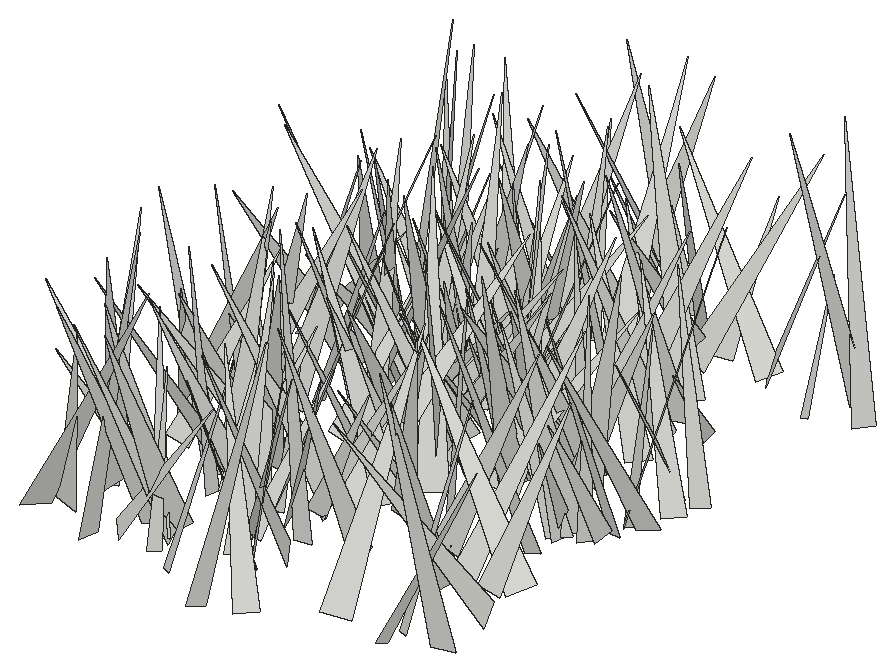
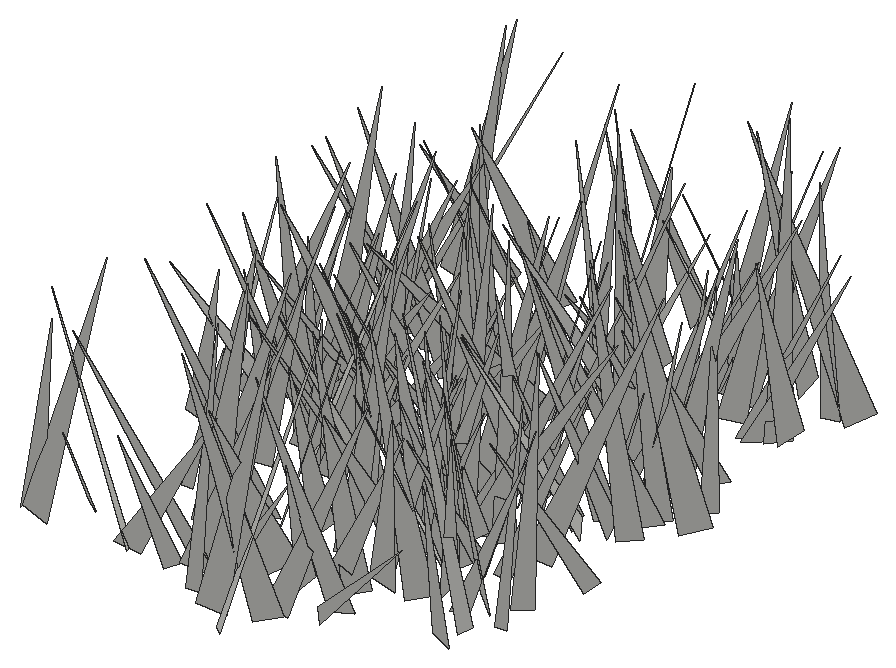
# SketchUp Ruby script. Lengths in inches.
U = 1.inch
M = Sketchup.active_model
def pt(a) = Geom::Point3d.new(a.map { |v| v * U })
def face(e, loops, mat)
  f = e.add_face(loops[0].map { |a| pt(a) })
  loops[1..].each { |l| e.add_face(l.map { |a| pt(a) }).erase! }
  f.material = f.back_material = mat if mat
  f
end
# faces: each face lists its corners as indices into pts; further lists are holes
def faces(e, pts, list, mat = nil) = list.each { |f| face(e, (f[0].is_a?(Array) ? f : [f]).map { |l| l.map { |i| pts[i] } }, mat) }
# xy, xz, yz: faces in a plane at the given z, y or x. An outline is a flat list of corners, or four numbers for a rectangle; further outlines are holes
def ring(l) = l.size == 4 ? [[l[0], l[1]], [l[2], l[1]], [l[2], l[3]], [l[0], l[3]]] : l.each_slice(2).to_a
def flat(e, list, mat, &to3) = list.each { |f| face(e, (f[0].is_a?(Array) ? f : [f]).map { |l| ring(l).map { |u, v| to3.(u, v) } }, mat) }
def xy(e, z, list, mat = nil) = flat(e, list, mat) { |x, y| [x, y, z] }
def xz(e, y, list, mat = nil) = flat(e, list, mat) { |x, z| [x, y, z] }
def yz(e, x, list, mat = nil) = flat(e, list, mat) { |y, z| [x, y, z] }
def lines(e, pts, list) = list.each { |a, b| e.add_line(pt(pts[a]), pt(pts[b])) }
# prism: a flat outline (further loops are holes) pulled along v
def prism(e, loops, v, mat = nil)
  f = face(e, loops, mat); d = Geom::Vector3d.new(v.map { |x| x * U })
  f.pushpull(f.normal.samedirection?(d) ? d.length : -d.length)
end
def box(e, o, s, mat = nil) = prism(e, [[o, [o[0] + s[0], o[1], o[2]], [o[0] + s[0], o[1] + s[1], o[2]], [o[0], o[1] + s[1], o[2]]]], [0, 0, s[2]], mat)
def at(x, y, z, deg = 0) = Geom::Transformation.translation(pt([x, y, z])) * Geom::Transformation.rotation(ORIGIN, Z_AXIS, deg.degrees)
def axes(o, x, y, z) = Geom::Transformation.new([*x, 0, *y, 0, *z, 0, *pt(o).to_a, 1])
def part(name) = M.definitions.add(name)
# library, detail: a bought-in or finely detailed component or shape, given as its bounding box
def library(name, o, s) = part(name).tap { |d| box(d.entities, o, s) }
def detail(e, o, s) = box(e.add_group.entities, o, s)
def put(e, d, t, mat = nil) = e.add_instance(d, t).tap { |i| i.material = mat if mat }
def group(e, t, mat = nil) = e.add_group.tap { |g| g.transformation = t; g.material = mat if mat }.entities
root = M.entities
c1 = part("fur_instance\#9")
p = [[0.8125,0,1.79],[0.67,-0.02,1.48],[0,-0.11,0],[0,0.11,0]]
faces(c1.entities,p,[[0,1,2,3]])
put(root,c1,axes([478.73,175.67,-21.66],[-5.72955,1.74546,0.28048],[1.75274,5.48455,1.67353],[-0.23061,-1.68113,5.75097]))
put(root,c1,axes([477.37,174.2,-21.66],[-6.45449,2.84921,1.13675],[2.42101,6.35763,-2.18855],[1.88385,1.59157,6.70736]))
put(root,c1,axes([478.21,201.08,-21.66],[1.19098,5.93826,0.851],[5.76454,-1.37303,1.51343],[-1.66049,-0.50738,5.86438]))
put(root,c1,axes([475.85,182.62,-21.66],[5.48383,-1.63022,0.30334],[-1.45467,-5.23263,-1.82362],[-0.79597,-1.66854,5.42259]))
put(root,c1,axes([476.59,198.27,-21.66],[-1.94792,-5.41513,0.85515],[-5.11405,2.12183,1.78705],[1.97517,0.15336,5.47032]))
put(root,c1,axes([479.69,182.78,-21.66],[-6.30755,-1.0303,0.95825],[-1.23667,6.15876,-1.51833],[0.67114,1.66527,6.20817]))
put(root,c1,axes([479.28,198.21,-21.66],[-4.32688,2.05759,1.06704],[2.30248,4.07514,1.47851],[0.2661,-1.80382,4.55737]))
put(root,c1,axes([478.76,196.84,-21.66],[4.06044,6.49572,1.60929],[6.19974,-4.35997,1.95581],[-2.5194,-0.26008,7.4065]))
put(root,c1,axes([479.375,175.64,-21.66],[-5.28354,-0.86585,0.73138],[-0.45173,4.80676,2.42722],[1.0395,-2.31209,4.77222]))
put(root,c1,axes([480.05,179.39,-21.66],[-1.59145,-6.67923,2.98055],[-7.18236,0.85085,-1.92829],[-1.38185,3.26993,6.58988]))
put(root,c1,axes([476.96,196.1,-21.66],[6.03542,-2.39463,0.80521],[-2.12324,-5.9379,-1.74415],[-1.3691,-1.34759,6.25448]))
put(root,c1,axes([475.61,192.22,-21.66],[3.92135,-2.35365,0.03406],[-2.05535,-3.39138,2.27856],[1.14733,1.96892,3.96545]))
put(root,c1,axes([477.05,171.45,-21.66],[-0.17668,-5.97479,1.5156],[-5.97573,0.53792,1.42395],[1.51188,1.4279,5.80532]))
put(root,c1,axes([479.55,191.72,-21.66],[4.2838,-6.03866,0.74714],[-5.20831,-4.11147,-3.36808],[-3.14598,-1.41597,6.59337]))
put(root,c1,axes([475.19,184.5,-21.66],[4.73655,-6.32836,0.37656],[-6.13582,-4.45802,2.25891],[1.59428,1.644,7.57499]))
put(root,c1,axes([481.03,193.74,-21.66],[-5.46466,-2.11839,0.66349],[-2.21236,5.05235,-2.09036],[-0.18243,2.18553,5.47545]))
put(root,c1,axes([477.65,174.89,-21.66],[7.83218,-2.47016,1.5817],[-2.12062,-7.88445,-1.81244],[-2.02643,-1.29626,8.00998]))
put(root,c1,axes([478.59,186.95,-21.66],[5.94248,2.0649,1.47313],[1.51819,-5.90154,2.14801],[-2.032,1.62942,5.91295]))
put(root,c1,axes([481.06,196.81,-21.66],[-6.67208,0.88571,0.68005],[0.61302,6.34873,-2.25421],[0.93335,2.16166,6.3419]))
put(root,c1,axes([477.32,180,-21.66],[-0.99691,5.86129,1.26655],[5.41282,1.43213,-2.36709],[2.58075,-0.73958,5.45394]))
put(root,c1,axes([479.28,183.15,-21.66],[5.03177,-2.92165,1.14225],[-2.20313,-4.82824,-2.64459],[-2.23316,-1.81978,5.18275]))
put(root,c1,axes([477.25,184.72,-21.66],[0.83878,-6.84447,1.51714],[-6.71971,-0.34936,2.13903],[1.99848,1.69801,6.55552]))
put(root,c1,axes([477.18,187.3,-21.66],[2.07111,-6.85146,1.31632],[-6.80663,-1.68294,1.94991],[1.53132,1.78604,6.88693]))
put(root,c1,axes([475.84,170.59,-21.66],[7.56022,-3.29271,0.03526],[-3.23696,-7.41517,1.59297],[0.60437,1.47429,8.09082]))
put(root,c1,axes([481.2,182.07,-21.66],[-6.30471,-1.37126,0.42808],[-1.05468,5.72683,2.8114],[0.97532,-2.67133,5.80738]))
put(root,c1,axes([484.07,190.01,-21.66],[-5.6206,-6.05261,0.8091],[-5.56666,4.62654,-4.06048],[-2.5102,3.29256,7.1929]))
put(root,c1,axes([479.79,194.22,-21.66],[4.40481,-2.70951,0.82389],[-1.71706,-3.76665,-3.20728],[-2.2521,-2.42766,4.05674]))
put(root,c1,axes([481.92,178.79,-21.66],[-0.45254,-7.13046,0.09555],[-6.72101,0.39447,-2.39372],[-2.38342,0.24148,6.7319]))
put(root,c1,axes([481.65,182.78,-21.66],[-4.16837,-0.36819,0.02902],[-0.35612,3.91965,-1.4217],[-0.09791,1.41863,3.93569]))
put(root,c1,axes([477.19,185.42,-21.66],[0.42432,7.03314,2.02201],[6.63788,0.48281,-3.07232],[3.08094,-2.00885,6.34082]))
put(root,c1,axes([479.92,169.64,-21.66],[-7.4216,0.05563,3.73189],[-0.80703,8.0859,-1.72548],[3.64401,1.90407,7.21845]))
put(root,c1,axes([482.03,176.91,-21.66],[-6.19983,-0.76734,1.02255],[-1.02443,6.01091,-1.70052],[0.76483,1.83095,6.01123]))
put(root,c1,axes([481.72,172.77,-21.66],[0.79588,-7.21699,0.96951],[-7.03929,-1.01213,-1.75565],[-1.86367,0.74092,7.04528]))
put(root,c1,axes([480.85,174.63,-21.66],[4.14575,-5.15062,1.64406],[-4.88287,-4.45639,-1.64839],[-2.32151,0.17524,6.40304]))
put(root,c1,axes([483.37,191.71,-21.66],[-7.87957,1.88276,1.17896],[2.17634,7.41366,2.70618],[0.44527,-2.91806,7.63603]))
put(root,c1,axes([480.29,187.55,-21.66],[4.99403,0.89918,1.35491],[0.3935,-4.91429,1.81096],[-1.5778,1.62046,4.74018]))
put(root,c1,axes([477.8125,199.6,-21.66],[8.03575,1.73258,0.69022],[1.85682,-7.7181,-2.24381],[-0.17451,-2.34107,7.90825]))
put(root,c1,axes([481.43,178.94,-21.66],[-6.63675,3.07759,1.929],[2.57186,6.8191,-2.03087],[2.56478,1.12578,7.02806]))
put(root,c1,axes([479.83,187.86,-21.66],[6.02604,4.35688,0.13616],[4.14402,-5.7981,2.12678],[-1.35204,1.64734,7.12547]))
put(root,c1,axes([479.25,186.46,-21.66],[0.24663,7.62872,2.41582],[7.70784,0.42293,-2.12242],[2.15005,-2.39126,7.33168]))
put(root,c1,axes([482.8125,171.75,-21.66],[0.07199,5.81915,0.58708],[5.58747,-0.24194,1.7129],[-1.72841,-0.53974,5.5618]))
put(root,c1,axes([484.52,202.88,-21.66],[-3.03964,-3.22245,0.08473],[-2.53096,2.3136,-2.80576],[-1.9964,1.97328,3.42802]))
put(root,c1,axes([482.71,178.54,-21.66],[-6.34287,-0.8603,1.40577],[-0.30586,6.10717,2.3574],[1.61949,-2.21602,5.95103]))
put(root,c1,axes([483.16,172.38,-21.66],[-6.61379,-2.13915,0.88077],[-1.88588,6.53057,1.69974],[1.33985,-1.36736,6.74011]))
put(root,c1,axes([482.19,194.6,-21.66],[-7.10447,-2.39928,3.44832],[-3.25719,7.42464,-1.54476],[2.65295,2.69055,7.33783]))
put(root,c1,axes([483.21,187.4,-21.66],[0.69074,-4.72184,2.34998],[-4.89788,-1.45354,-1.48096],[-1.95676,1.97148,4.53648]))
put(root,c1,axes([481.4,193.74,-21.66],[4.67368,1.9817,0.84614],[1.46066,-4.3994,2.23565],[-1.58416,1.79011,4.55767]))
put(root,c1,axes([483.39,193.12,-21.66],[0.65103,4.23875,0.31259],[3.78552,-0.72206,1.9071],[-1.9325,0.01355,3.84107]))
put(root,c1,axes([484.04,198.4375,-21.66],[-0.66678,7.09806,0.59701],[6.83624,0.46921,2.05647],[-2.00116,-0.76214,6.82627]))
put(root,c1,axes([482.55,177.52,-21.66],[-4.05374,2.9207,0.15477],[2.65047,3.78022,-1.91631],[1.23673,1.47198,4.61422]))
put(root,c1,axes([484.17,186.86,-21.66],[-2.33068,3.85921,0.35584],[3.66264,2.05758,1.6744],[-1.26695,-1.15111,4.18592]))
put(root,c1,axes([484.62,190.7,-21.66],[-2.52034,-4.28654,0.32351],[-4.12689,2.30776,-1.57296],[-1.20326,1.06349,4.71724]))
put(root,c1,axes([483.43,170.51,-21.66],[-4.4668,1.24969,0.75909],[0.98308,4.37301,-1.41442],[1.08236,1.18546,4.4174]))
put(root,c1,axes([481.94,194.45,-21.66],[4.14579,-2.60609,2.17076],[-3.31381,-3.84297,1.71517],[-0.72292,2.67047,4.58667]))
put(root,c1,axes([484.58,197.85,-21.66],[-5.48359,2.23586,1.70204],[2.68404,5.27249,1.72124],[0.83185,-2.27324,5.66623]))
put(root,c1,axes([483.03,172.86,-21.66],[6.13444,-4.45258,1.42838],[-3.84619,-6.14459,-2.6359],[-2.65943,-1.38408,7.10696]))
put(root,c1,axes([483.26,191.9375,-21.66],[-5.22484,3.83291,1.4033],[3.4058,5.3502,-1.93269],[2.24967,0.80218,6.18505]))
put(root,c1,axes([484.76,194.11,-21.66],[-1.35927,-4.19334,1.10265],[-4.18909,0.97193,-1.4678],[-1.11869,1.45561,4.1566]))
put(root,c1,axes([483.79,187.77,-21.66],[-5.87667,-3.9224,1.1719],[-3.54254,5.90008,1.98324],[2.05159,-1.04767,6.78139]))
put(root,c1,axes([486.01,199.73,-21.66],[-1.67581,5.69721,1.32161],[5.39716,0.9769,2.63242],[-2.25291,-1.89755,5.32325]))
put(root,c1,axes([481.97,191.34,-21.66],[7.49694,-1.26912,1.50095],[-0.87324,-7.45265,-1.93987],[-1.76095,-1.70734,7.35199]))
put(root,c1,axes([484.94,177.05,-21.66],[-5.93651,2.05948,0.4431],[1.83167,5.70073,-1.95618],[1.04056,1.71471,5.97135]))
put(root,c1,axes([483.36,194.67,-21.66],[4.16098,5.56887,0.17793],[5.30628,-4.02846,1.99315],[-1.69922,1.05685,6.65984]))
put(root,c1,axes([482.3,178.57,-21.66],[0.05703,4.78722,0.58826],[4.57544,0.13244,-1.52137],[1.52606,-0.57598,4.5394]))
put(root,c1,axes([480.63,171.08,-21.66],[4.14208,3.82367,0.06036],[3.46383,-3.71363,-2.44781],[1.62049,-1.8356,5.07794]))
put(root,c1,axes([485.13,185.625,-21.66],[-7.34828,2.49323,1.09592],[2.03506,7.1224,-2.5582],[1.80991,2.11416,7.32591]))
put(root,c1,axes([481.69,198.39,-21.66],[3.71453,-6.09838,0.78607],[-6.05056,-3.46164,1.73599],[1.09493,1.55972,6.92635]))
put(root,c1,axes([484.27,194.93,-21.66],[6.50516,0.09741,3.11354],[0.81371,-7.01185,-1.48071],[-3.00691,-1.68675,6.33514]))
put(root,c1,axes([486.62,180.375,-21.66],[-7.42366,-0.80204,0.92134],[-0.52005,7.2098,2.08597],[1.1053,-1.9946,7.16957]))
put(root,c1,axes([483.36,185.23,-21.66],[-0.37436,5.47936,0.25355],[5.20879,0.43477,-1.70506],[1.71934,-0.12411,5.22075]))
put(root,c1,axes([482.33,180.87,-21.66],[2.66865,-7.95792,0.14871],[-7.80747,-2.5868,1.68053],[1.54726,0.67254,8.22351]))
put(root,c1,axes([486.47,203.86,-21.66],[1.14957,-5.99203,1.40359],[-5.68779,-1.57972,-2.08556],[-2.35023,0.89221,5.73379]))
put(root,c1,axes([485.45,184.5,-21.66],[-4.40501,-3.46188,0.56585],[-3.18391,4.32713,1.68747],[1.47225,-1.00011,5.34239]))
put(root,c1,axes([483.33,194.55,-21.66],[0.81031,-5.69395,0.84212],[-5.55553,-0.55126,1.61834],[1.50543,1.03047,5.51893]))
put(root,c1,axes([485.77,177.46,-21.66],[-3.80527,0.70423,0.62745],[0.3357,3.44844,-1.83447],[0.88144,1.72686,3.40746]))
put(root,c1,axes([485.15,169.33,-21.66],[3.44077,4.42208,0.21812],[4.18127,-3.33634,1.68138],[-1.45578,0.8691,5.34478]))
put(root,c1,axes([486.83,191.67,-21.66],[-7.37463,3.18086,0.67882],[2.84062,7.11825,-2.49505],[1.58417,2.04365,7.63399]))
put(root,c1,axes([486.42,191.14,-21.66],[-4.94323,1.53486,1.76986],[2.06825,4.80019,1.61379],[1.10026,-2.12747,4.91803]))
put(root,c1,axes([483.8,201.93,-21.66],[-0.17372,7.00266,1.70424],[6.95108,0.61311,-1.81067],[1.90374,-1.5996,6.76675]))
put(root,c1,axes([482.94,187.25,-21.66],[8.11647,0.24258,0.67526],[0.10402,-7.98511,1.61836],[-0.70993,1.60345,7.95719]))
put(root,c1,axes([486.875,172.78,-21.66],[-6.53703,2.92768,0.70077],[2.53956,6.26275,-2.47462],[1.61648,2.00045,6.72163]))
put(root,c1,axes([486.96,200.8,-21.66],[-5.33411,1.7362,0.45715],[1.45522,5.02033,-2.08679],[1.05153,1.85957,5.20696]))
put(root,c1,axes([489.61,187.03,-21.66],[-2.20634,6.02099,1.75888],[5.48729,0.94934,3.63349],[-3.03901,-2.65713,5.28374]))
put(root,c1,axes([484.9,191.16,-21.66],[7.37439,-3.31849,1.28024],[-2.90244,-7.31769,-2.24953],[-2.05603,-1.57231,7.76747]))
put(root,c1,axes([488.52,172.29,-21.66],[-3.99392,-3.16377,0.39905],[-3.06383,3.62986,-1.88605],[-0.88412,1.71311,4.73326]))
put(root,c1,axes([486.43,194.28,-21.66],[-4.56686,4.07542,0.09193],[3.68922,4.19072,-2.51023],[1.73411,1.8173,5.58247]))
put(root,c1,axes([489.04,191.51,-21.66],[-3.06534,4.86368,0.18481],[4.51167,2.75744,2.26433],[-1.82603,-1.35165,5.28436]))
put(root,c1,axes([485.63,177.1875,-21.66],[6.81061,4.1437,0.72104],[3.52808,-6.3754,3.31382],[-2.28972,2.50169,7.25074]))
put(root,c1,axes([488.65,175.82,-21.66],[1.70019,7.5386,2.42367],[7.33263,-2.43467,2.42902],[-2.9895,-1.68439,7.33628]))
put(root,c1,axes([486.35,174.67,-21.66],[-3.43381,3.18637,0.41007],[2.54254,3.06224,-2.50406],[1.96382,1.60682,3.959]))
put(root,c1,axes([485.68,192.21,-21.66],[4.75134,-2.11282,0.36953],[-1.90852,-4.57438,-1.61505],[-0.97883,-1.33672,4.94275]))
put(root,c1,axes([487.5,207.17,-21.66],[-5.6893,-5.57398,0.54513],[-5.22917,5.56506,2.3282],[2.00554,-1.30211,7.61688]))
put(root,c1,axes([488.46,193.91,-21.66],[-5.41908,-0.82486,1.13145],[-1.12996,5.24719,-1.58656],[0.82691,1.76453,5.24687]))
put(root,c1,axes([484.43,199.91,-21.66],[3.61715,-5.66391,0.01487],[-5.50634,-3.51236,1.58351],[1.3268,0.86448,6.53117]))
put(root,c1,axes([489.6,181.55,-21.66],[-4.16416,5.80884,2.0419],[6.1268,3.66414,2.07088],[-0.6118,-2.84317,6.84063]))
put(root,c1,axes([488.38,184.23,-21.66],[2.87814,-5.28951,1.31735],[-4.95416,-3.15966,-1.86304],[-2.27391,0.18887,5.72641]))
put(root,c1,axes([486.94,186.61,-21.66],[5.11337,-4.37567,0.02712],[-4.08728,-4.79107,-2.37351],[-1.56248,-1.78687,6.29758]))
put(root,c1,axes([489.11,205.72,-21.66],[1.07794,-7.21694,3.00432],[-7.53412,-1.768,-1.54384],[-2.08502,2.65746,7.13181]))
put(root,c1,axes([490.07,204.28,-21.66],[-2.15609,-3.98258,0.83043],[-3.73233,1.56246,-2.1972],[-1.61872,1.70208,3.96005]))
put(root,c1,axes([485.15,187.94,-21.66],[4.61387,-2.10989,0.31356],[-1.93342,-3.82099,2.73855],[0.90102,2.60502,4.2708]))
put(root,c1,axes([488.56,189.28,-21.66],[3.46257,-3.0651,1.27719],[-2.41097,-3.5895,-2.07802],[-2.28326,-0.85797,4.13111]))
put(root,c1,axes([488.94,200.15,-21.66],[-6.13074,4.86156,0.06985],[4.48302,5.69573,-2.94734],[1.88206,2.26926,7.24803]))
put(root,c1,axes([487.48,196.88,-21.66],[7.10031,-2.91459,1.55919],[-2.29482,-7.00551,-2.64516],[-2.37902,-1.94118,7.20502]))
put(root,c1,axes([489.1875,191.72,-21.66],[2.9038,6.51052,1.10748],[6.2299,-3.10193,1.9005],[-2.1913,-0.1914,6.87074]))
put(root,c1,axes([486.22,204.77,-21.66],[3.6811,-6.05089,2.6185],[-6.53456,-2.94932,2.37094],[0.87715,3.42178,6.67401]))
put(root,c1,axes([490.92,168.46,-21.66],[-1.83761,6.5724,0.07775],[6.30696,1.74042,1.94227],[-1.85059,-0.59481,6.54223]))
put(root,c1,axes([490.53,183.8,-21.66],[-7.32021,3.8589,0.48336],[3.73123,7.2592,-1.44642],[1.09666,1.05977,8.14767]))
put(root,c1,axes([491.01,185.98,-21.66],[-4.07281,-4.5818,0.7427],[-4.55178,3.7491,-1.83244],[-0.90871,1.75604,5.85003]))
put(root,c1,axes([488.79,174.46,-21.66],[-6.12859,-4.53414,1.24355],[-3.97845,6.08997,2.59781],[2.50535,-1.42065,7.16724]))
put(root,c1,axes([488.52,167.48,-21.66],[6.48387,0.57283,2.72889],[-0.5216,-6.53637,2.61139],[-2.73914,2.60063,5.96233]))
put(root,c1,axes([489.72,196.06,-21.66],[-6.30964,2.41528,1.06239],[1.96226,6.1361,-2.29599],[1.76402,1.81341,6.35402]))
put(root,c1,axes([490.02,192.22,-21.66],[-5.70534,2.42628,0.74712],[2.22137,5.6608,-1.42016],[1.22905,1.03174,6.03498]))
put(root,c1,axes([488.65,191.41,-21.66],[-3.02452,-1.82217,1.01563],[-1.34667,3.07159,1.50047],[1.5932,-0.86291,3.19635]))
put(root,c1,axes([486.71,173.78,-21.66],[6.48852,0.93317,0.66882],[1.0636,-6.33108,-1.48501],[-0.43231,-1.57025,6.38486]))
put(root,c1,axes([490.43,192.22,-21.66],[-4.5545,1.12209,0.15618],[1.0267,4.36161,-1.39615],[0.47894,1.3207,4.4781]))
put(root,c1,axes([486.59,177.43,-21.66],[6.70588,0.95076,0.50826],[1.07552,-6.12086,-2.74035],[-0.07444,-2.78609,6.19381]))
put(root,c1,axes([492.1,196.14,-21.66],[-6.74391,-2.32387,0.77011],[-2.44649,6.31426,-2.37034],[-0.09,2.49068,6.72772]))
put(root,c1,axes([487.33,178.54,-21.66],[1.64693,-4.65446,0.85777],[-4.4282,-1.19483,2.01879],[1.67056,1.42146,4.50564]))
put(root,c1,axes([486.68,191.4,-21.66],[3.67258,4.04026,0.63824],[3.75616,-2.99162,-2.6759],[1.61937,-2.22383,4.75932]))
put(root,c1,axes([485.88,189.38,-21.66],[4.06376,5.39951,0.02576],[4.83357,-3.62337,-3.0294],[2.40665,-1.8401,6.04083]))
put(root,c1,axes([488.38,172.04,-21.66],[5.36268,3.16176,1.79895],[3.56295,-5.21159,-1.4615],[-0.73371,-2.1986,6.05138]))
put(root,c1,axes([487.64,184.19,-21.66],[2.89446,-5.47209,0.08006],[-5.31049,-2.7865,1.53693],[1.32243,0.78724,5.99662]))
put(root,c1,axes([487.96,180.17,-21.66],[-4.06981,7.2471,0.38585],[5.9474,3.58401,-4.58433],[4.15906,1.9665,6.9331]))
put(root,c1,axes([493.17,190.29,-21.66],[-4.54236,-5.48641,0.31776],[-5.31376,4.27953,-2.06985],[-1.40202,1.55551,6.81539]))
put(root,c1,axes([487.24,178.86,-21.66],[3.70489,5.29932,0.63458],[5.07029,-3.25343,-2.43293],[1.66665,-1.88258,5.99082]))
put(root,c1,axes([489.51,185.78,-21.66],[6.5233,2.37968,3.04495],[3.30026,-6.53866,-1.96019],[-2.01069,-3.01183,6.66138]))
put(root,c1,axes([490.35,182.79,-21.66],[-3.99829,-3.957,0.07334],[-3.50173,3.58563,2.55553],[1.84422,-1.77059,5.01133]))
put(root,c1,axes([489.37,191.8,-21.66],[5.91646,3.40669,0.5347],[3.12979,-5.75065,2.00759],[-1.44773,1.49011,6.52531]))
put(root,c1,axes([487.25,193.24,-21.66],[2.23337,6.49328,0.05356],[5.9184,-2.0122,-2.84202],[2.67172,-0.9705,6.25089]))
put(root,c1,axes([492.19,190.23,-21.66],[0.25275,3.74041,1.98428],[3.79537,-1.08135,1.55493],[-1.87703,-1.68284,3.41127]))
put(root,c1,axes([493.41,187.68,-21.66],[-0.91918,-4.72146,0.08029],[-4.18667,0.777,-2.23865],[-2.18412,0.49761,4.25741]))
put(root,c1,axes([492.07,176.34,-21.66],[-7.41474,-1.37074,2.09218],[-0.74138,7.45582,2.25736],[2.38883,-1.94072,7.19456]))
put(root,c1,axes([488.17,186.14,-21.66],[4.70359,-4.43483,0.77561],[-4.1988,-3.91632,3.07011],[1.62462,2.71804,5.6891]))
put(root,c1,axes([493.7,188.19,-21.66],[-0.77186,4.35622,1.72795],[4.2436,-0.09339,2.13104],[-1.98854,-1.8902,3.87699]))
put(root,c1,axes([492.8,191.58,-21.66],[2.20766,-6.15742,1.48059],[-5.96151,-2.54967,-1.71445],[-2.13691,0.75174,6.31254]))
put(root,c1,axes([492.41,203.03,-21.66],[3.27442,-5.47757,0.11686],[-5.10679,-3.10069,-2.24625],[-1.98447,-1.05885,5.97327]))
put(root,c1,axes([491.02,204.76,-21.66],[-2.08812,-6.42397,1.05341],[-6.15561,2.30841,1.87538],[2.11792,0.37569,6.48927]))
put(root,c1,axes([492.36,186.7,-21.66],[3.62911,6.60842,0.2466],[6.35712,-3.56375,1.94657],[-1.82181,0.72867,7.28371]))
put(root,c1,axes([490.99,191.56,-21.66],[5.45875,-2.61976,0.1584],[-2.41646,-5.15945,-2.05595],[-1.02417,-1.78972,5.6951]))
put(root,c1,axes([496.28,203.44,-21.66],[-3.37764,5.82202,0.02709],[5.22944,3.02002,2.9728],[-2.55923,-1.51283,6.03878]))
put(root,c1,axes([490.9,188.48,-21.66],[1.63148,3.88333,0.8996],[3.80186,-1.22375,-1.61232],[1.19808,-1.40479,3.89132]))
put(root,c1,axes([494.57,199.09,-21.66],[-3.07753,7.46975,2.03134],[7.70521,2.74591,1.57617],[-0.74375,-2.46119,7.92363]))
put(root,c1,axes([494.6,197.09,-21.66],[-1.73609,5.26171,0.91511],[5.1615,1.40586,1.70864],[-1.37182,-1.3693,5.27069]))
put(root,c1,axes([494.61,190.79,-21.66],[1.00631,5.78428,1.17144],[5.41169,-1.37849,2.15781],[-2.35451,-0.6962,5.46025]))
put(root,c1,axes([494.09,191.9,-21.66],[-5.79035,-4.99721,0.36352],[-4.82955,5.71454,1.62848],[1.33407,-1.00217,7.47317]))
put(root,c1,axes([491.06,180.92,-21.66],[0.69431,-7.1025,1.01226],[-6.95299,-0.41552,1.85354],[1.7681,1.15502,6.89145]))
put(root,c1,axes([493.24,186.7,-21.66],[-5.97447,-2.65496,2.2585],[-2.10106,6.3191,1.8704],[2.78122,-0.92951,6.26456]))
put(root,c1,axes([494.42,180.11,-21.66],[3.23969,5.31398,1.47982],[4.81259,-3.56155,2.25346],[-2.69577,0.02794,5.80137]))
put(root,c1,axes([497.41,185.34,-21.66],[-2.18408,5.95276,0.46734],[5.01759,1.55993,3.57972],[-3.2369,-1.59851,5.23366]))
put(root,c1,axes([493.32,203.47,-21.66],[-2.78361,3.37072,1.19614],[3.02117,3.0272,-1.49988],[1.91443,0.12385,4.10617]))
put(root,c1,axes([495.82,197.12,-21.66],[-1.13695,-6.80591,1.9758],[-6.92615,0.64332,-1.76957],[-1.50086,2.18691,6.66945]))
put(root,c1,axes([494.23,190.11,-21.66],[6.48177,-5.01878,0.45242],[-4.24735,-5.8379,-3.90962],[-2.71162,-2.85253,7.2053]))
put(root,c1,axes([493.49,186.53,-21.66],[7.48346,-2.4752,1.75576],[-1.96533,-7.51292,-2.21472],[-2.31232,-1.62508,7.56464]))
put(root,c1,axes([494.61,188.47,-21.66],[2.5877,-3.76016,0.15432],[-3.53923,-2.49522,-1.45139],[-1.27925,-0.70276,4.32764]))
put(root,c1,axes([494.63,170.96,-21.66],[-5.35866,5.61511,0.59327],[5.12673,5.1813,-2.73266],[2.36603,1.4904,7.2648]))
put(root,c1,axes([496.56,192.67,-21.66],[-3.37701,5.49526,1.43426],[5.6473,3.0721,1.52623],[-0.60248,-2.00587,6.26679]))
put(root,c1,axes([496.47,195.05,-21.66],[-7.7703,-1.5883,1.42664],[-1.2052,7.70803,2.01725],[1.76224,-1.7318,7.67014]))
put(root,c1,axes([493.1,186.125,-21.66],[-3.36255,6.42423,2.20976],[5.77924,4.00105,-2.8377],[3.57129,-0.42595,6.67271]))
put(root,c1,axes([495.81,190.13,-21.66],[2.24091,-5.47361,0.67385],[-5.23088,-2.33999,-1.61199],[-1.7471,-0.01469,5.69066]))
put(root,c1,axes([492.25,186.38,-21.66],[0.90469,6.24799,0.05202],[5.52251,-0.775,-2.9597],[2.92267,-0.46962,5.57638]))
put(root,c1,axes([492.68,196.66,-21.66],[1.48421,7.77893,1.22221],[7.56365,-1.06243,-2.42301],[2.19017,-1.60247,7.53948]))
put(root,c1,axes([492.47,202.27,-21.66],[1.86343,6.88556,0.79652],[6.51007,-1.45535,-2.64927],[2.37997,-1.41024,6.62304]))
put(root,c1,axes([498.29,182.09,-21.66],[-2.5015,-6.23633,1.72664],[-6.18785,1.76379,-2.59425],[-1.89304,2.47545,6.19832]))
put(root,c1,axes([500.24,178.74,-21.66],[-5.51381,4.9525,0.02994],[4.6746,5.18943,2.47955],[-1.63592,-1.86355,6.98435]))
put(root,c1,axes([494.23,190.41,-21.66],[3.12045,6.97557,0.92804],[6.87353,-2.80376,-2.03727],[1.5081,-1.6545,7.36514]))
put(root,c1,axes([498.33,184.13,-21.66],[-3.08305,4.83073,2.80211],[5.58378,2.72141,1.452],[0.09585,-3.15451,5.54372]))
put(root,c1,axes([494.52,179.82,-21.66],[2.05152,-6.6713,2.37008],[-6.64568,-0.96384,3.03943],[2.44098,2.98279,6.28306]))
put(root,c1,axes([496.09,189.14,-21.66],[2.2039,-6.87435,1.74953],[-7.02125,-1.85328,1.56272],[1.00974,2.1174,7.04782]))
put(root,c1,axes([495.41,189.35,-21.66],[3.73995,-4.97965,1.07609],[-4.97131,-3.27521,2.12161],[1.114,2.10195,5.85517]))
put(root,c1,axes([496.97,176.26,-21.66],[6.98894,-3.62557,1.01436],[-3.15649,-6.80873,-2.58782],[-2.05189,-1.87497,7.43594]))
put(root,c1,axes([499.59,184.6,-21.66],[-6.16922,0.32467,1.04524],[-0.06119,5.87189,-2.18505],[1.09279,2.16166,5.77844]))
put(root,c1,axes([497.82,196.76,-21.66],[3.38324,-1.277,0.34003],[-0.90165,-2.91389,-1.97203],[-0.96612,-1.75247,3.03119]))
put(root,c1,axes([498.32,171.72,-21.66],[3.77258,4.9169,0.38845],[4.64704,-3.70729,1.79444],[-1.65279,0.7995,5.93196]))
put(root,c1,axes([498.55,184.5625,-21.66],[6.46231,-4.31648,2.52967],[-3.92803,-6.93665,-1.8017],[-3.09867,-0.20881,7.55958]))
put(root,c1,axes([500.3,186.0625,-21.66],[-2.82559,-5.19892,1.36333],[-5.31081,2.46391,-1.61114],[-0.82624,1.9421,5.69358]))
put(root,c1,axes([500.48,175.81,-21.66],[-7.29463,-2.71144,0.02018],[-2.47986,6.69465,3.09773],[1.09665,-2.89718,7.13916]))
put(root,c1,axes([496.91,178.43,-21.66],[1.06363,7.1406,0.14161],[6.98782,-1.01087,-1.51263],[1.47601,-0.35985,7.05914]))
put(root,c1,axes([496.22,203.39,-21.66],[5.98331,3.57339,0.75673],[3.63565,-5.68637,-1.89446],[0.35186,-2.00943,6.70672]))
put(root,c1,axes([498.28,184.86,-21.66],[4.1039,-1.37964,0.4984],[-1.03776,-3.77714,-1.91052],[-1.03675,-1.68037,3.88527]))
put(root,c1,axes([501.5,189.33,-21.66],[-1.94953,6.2532,0.70862],[6.08536,1.68405,1.8809],[-1.60411,-1.2111,6.27419]))
put(root,c1,axes([500.92,171.65,-21.66],[-1.04276,-7.37455,2.60053],[-7.71345,0.53914,-1.56404],[-1.28435,2.74945,7.28184]))
put(root,c1,axes([498.13,170.29,-21.66],[5.03908,0.51167,0.65236],[0.18588,-4.61324,2.18248],[-0.80798,2.12978,4.57066]))
put(root,c1,axes([500.16,187,-21.66],[5.94606,5.36025,0.59468],[4.2161,-5.17199,4.4628],[-3.36309,2.9933,6.64615]))
put(root,c1,axes([500.39,187.15,-21.66],[-4.99347,0.21503,1.45697],[-0.36457,4.80955,-1.95935],[1.42691,1.98134,4.59803]))
put(root,c1,axes([500.3,201.22,-21.66],[1.53322,3.39,0.04746],[3.12816,-1.43461,1.41479],[-1.30727,0.54307,3.44111]))
put(root,c1,axes([501.91,190.91,-21.66],[-0.60049,6.11637,0.8715],[5.86899,0.29123,2.00004],[-1.92986,-1.0175,5.81123]))
put(root,c1,axes([501.3,187.56,-21.66],[1.05272,-6.58483,0.46236],[-6.33643,-1.13928,-1.79827],[-1.85027,0.15508,6.42141]))
put(root,c1,axes([500.02,185.57,-21.66],[4.14247,-2.36814,0.94959],[-1.79033,-3.98803,-2.13546],[-1.81783,-1.46881,4.26707]))
put(root,c1,axes([502,203.68,-21.66],[-1.47229,-7.46087,2.3597],[-7.72207,0.99683,-1.66627],[-1.2659,2.59656,7.41996]))
put(root,c1,axes([503.14,202.4,-21.66],[-7.7657,1.30292,0.44128],[1.14319,7.51969,-2.08465],[0.76515,1.98873,7.59328]))
put(root,c1,axes([498.96,177.74,-21.66],[-0.64371,5.67181,1.6895],[5.48083,1.21245,-1.9821],[2.23257,-1.34117,5.35305]))
put(root,c1,axes([499.99,191.73,-21.66],[-3.50557,-5.51536,0.11612],[-4.95597,3.20905,2.80393],[2.42302,-1.41579,5.90306]))
